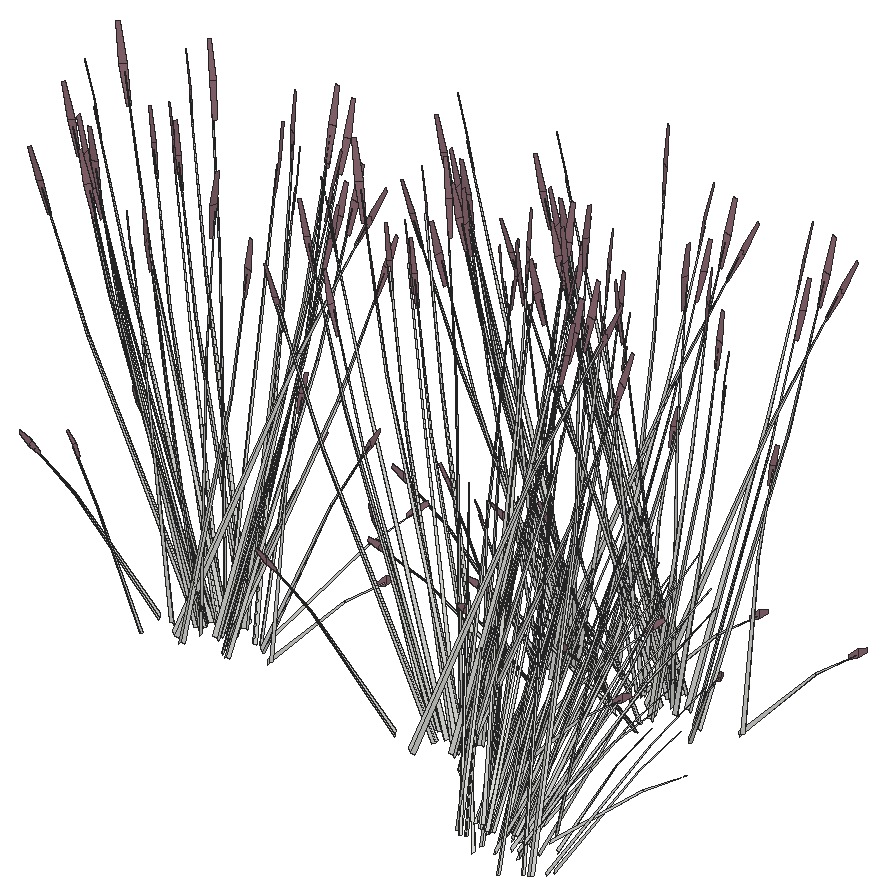
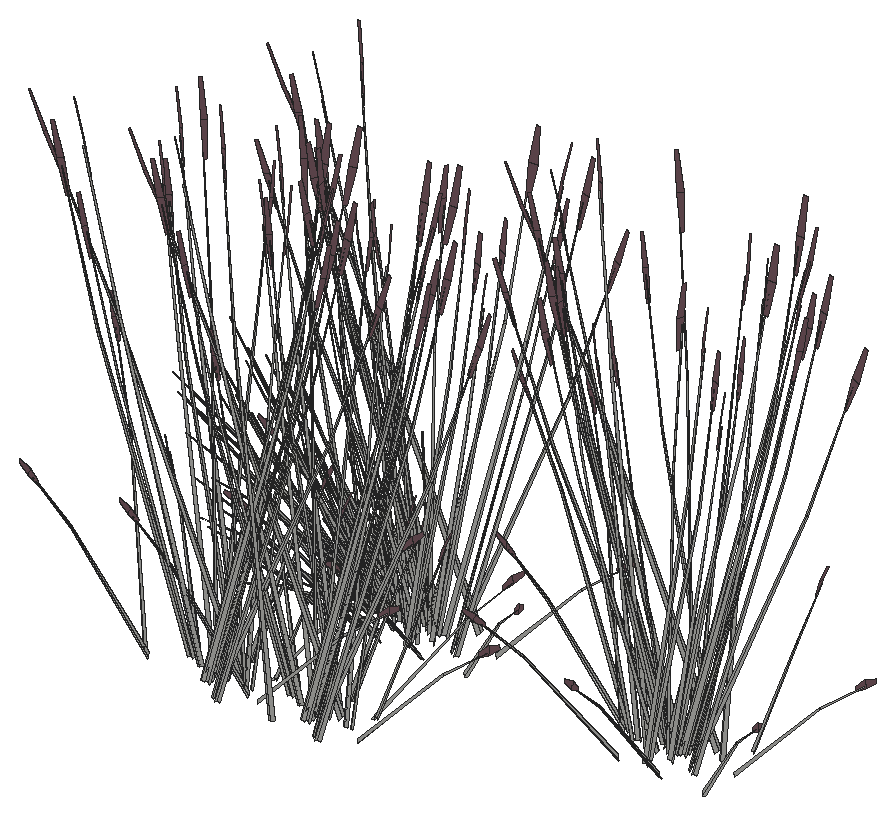
# SketchUp Ruby script. Lengths in inches.
U = 1.inch
M = Sketchup.active_model
def pt(a) = Geom::Point3d.new(a.map { |v| v * U })
def face(e, loops, mat)
  f = e.add_face(loops[0].map { |a| pt(a) })
  loops[1..].each { |l| e.add_face(l.map { |a| pt(a) }).erase! }
  f.material = f.back_material = mat if mat
  f
end
# faces: each face lists its corners as indices into pts; further lists are holes
def faces(e, pts, list, mat = nil) = list.each { |f| face(e, (f[0].is_a?(Array) ? f : [f]).map { |l| l.map { |i| pts[i] } }, mat) }
# xy, xz, yz: faces in a plane at the given z, y or x. An outline is a flat list of corners, or four numbers for a rectangle; further outlines are holes
def ring(l) = l.size == 4 ? [[l[0], l[1]], [l[2], l[1]], [l[2], l[3]], [l[0], l[3]]] : l.each_slice(2).to_a
def flat(e, list, mat, &to3) = list.each { |f| face(e, (f[0].is_a?(Array) ? f : [f]).map { |l| ring(l).map { |u, v| to3.(u, v) } }, mat) }
def xy(e, z, list, mat = nil) = flat(e, list, mat) { |x, y| [x, y, z] }
def xz(e, y, list, mat = nil) = flat(e, list, mat) { |x, z| [x, y, z] }
def yz(e, x, list, mat = nil) = flat(e, list, mat) { |y, z| [x, y, z] }
def lines(e, pts, list) = list.each { |a, b| e.add_line(pt(pts[a]), pt(pts[b])) }
# prism: a flat outline (further loops are holes) pulled along v
def prism(e, loops, v, mat = nil)
  f = face(e, loops, mat); d = Geom::Vector3d.new(v.map { |x| x * U })
  f.pushpull(f.normal.samedirection?(d) ? d.length : -d.length)
end
def box(e, o, s, mat = nil) = prism(e, [[o, [o[0] + s[0], o[1], o[2]], [o[0] + s[0], o[1] + s[1], o[2]], [o[0], o[1] + s[1], o[2]]]], [0, 0, s[2]], mat)
def at(x, y, z, deg = 0) = Geom::Transformation.translation(pt([x, y, z])) * Geom::Transformation.rotation(ORIGIN, Z_AXIS, deg.degrees)
def axes(o, x, y, z) = Geom::Transformation.new([*x, 0, *y, 0, *z, 0, *pt(o).to_a, 1])
def part(name) = M.definitions.add(name)
# library, detail: a bought-in or finely detailed component or shape, given as its bounding box
def library(name, o, s) = part(name).tap { |d| box(d.entities, o, s) }
def detail(e, o, s) = box(e.add_group.entities, o, s)
def put(e, d, t, mat = nil) = e.add_instance(d, t).tap { |i| i.material = mat if mat }
def group(e, t, mat = nil) = e.add_group.tap { |g| g.transformation = t; g.material = mat if mat }.entities
root = M.entities
M.materials.add("LightPink_Translucent").color = [144, 107, 117]
c1 = part("blade")
p = [[2.15,0.21,22],[0,0.17,0],[0.09,0.45,0],[2.18,0.31,22],[2.29,0.31,22],[0.38,0.45,0],
  [2.48,0.24,33],[2.49,0.24,33],[2.48,0.22,33]]
faces(c1.entities,p,[[0,1,2,3],[4,5,2,3],[6,3,4,7],[8,0,3,6]])
c2 = part("seeds")
p = [[0.3,-0.1,1.38],[-0.01,-0.03,1.59],[-0.01,-0.03,0.03],[0.14,-0.07,-0.07],[0.29,-0.03,3],[0.15,0.01,3.11]]
faces(c2.entities,p,[[0,1,2,3],[1,0,4,5]],"LightPink_Translucent")
c3 = part("blade with seeds")
put(c3.entities,c1,at(0,0,0))
put(c3.entities,c2,axes([2.4,0.25,30.99],[1.5799,-0.05474,1.17369],[-0.12525,1.92788,0.29478],[-0.07173,-0.02425,1.56792]))
c4 = part("blade with seeds\#1")
put(c4.entities,c1,at(0,0,0))
put(root,c3,axes([30.54,56.74,44.21],[0.59459,-0.93321,-0.44739],[1.23546,0.44912,0.21531],[0,-0.21512,1.43643]))
put(root,c3,axes([31.08,56.27,44.67],[-0.1428,-1.18174,-0.29095],[1.48733,-0.07145,-0.50002],[0.26191,-0.15741,1.59708]))
put(root,c4,axes([80.07,48.07,38.91],[-0.15413,-0.36483,1.28914],[0.46474,-0.90077,-0.27724],[0.40213,0.2681,0.55117]))
put(root,c3,axes([27.39,56.34,44.03],[0.85545,-0.64616,-0.30978],[0.85545,0.64616,0.30978],[0,-0.20813,1.38974]))
put(root,c3,axes([27.05,53.24,44.13],[-0.35352,0.84566,-0.03893],[-1.08806,-0.26014,-0.17649],[-0.1652,-0.13832,0.58215]))
put(root,c4,axes([71.29,48.59,38.49],[0.7978,0.33351,-0.03509],[-0.24541,1.02647,-0.15911],[-0.13049,0.15585,0.52479]))
put(root,c3,axes([61.53,54.7,44.06],[-1.27479,-0.1698,-0.62353],[0.26901,-1.04736,-0.16365],[-0.38043,-0.12691,1.37633]))
put(root,c3,axes([30.39,57.51,44.67],[-1.38012,-0.49416,-0.29095],[0.66454,-1.04299,-0.50002],[-0.04337,-0.25608,1.59708]))
put(root,c4,axes([76.27,48.65,41.13],[-0.13963,-1.00636,0.31925],[0.79822,-0.26574,-0.41216],[0.2144,0.28839,0.78863]))
put(root,c3,axes([30.88,53.66,44.03],[1.14332,0.25625,-0.30978],[-0.28787,0.90242,0.30978],[0.23049,-0.10406,1.38974]))
put(root,c3,axes([61.23,51.77,43.59],[-1.20625,0.41464,1.28929],[-0.38394,-1.1897,0.50096],[0.74071,0.01979,1.46642]))
put(root,c4,axes([78.54,50.93,41.66],[0.2608,-1.0202,-0.05849],[0.8027,0.31383,-0.26518],[0.12187,0.16686,0.87466]))
put(root,c4,axes([78.66,46.76,38.71],[0.97904,0.72283,0],[-0.54599,1.20931,-0.46523],[-0.12435,0.27543,1.47583]))
put(root,c4,axes([78.07,47.41,38.39],[-0.48852,1.08202,-0.44759],[-0.87598,-0.64674,0],[-0.11126,0.24644,1.41987]))
put(root,c3,axes([70.66,53.38,43.49],[-0.06405,-0.15723,1.76342],[0.44421,-0.91974,-0.26939],[0.4481,-0.01323,0.30037]))
put(root,c3,axes([57.43,53.22,43.49],[0.03108,0.16322,1.76342],[-0.62654,0.85237,-0.26939],[-0.44504,-0.04296,0.30037]))
put(root,c4,axes([71.57,45.96,41.0625],[-0.47225,0.98582,-0.64046],[-0.82754,-0.7006,0.07729],[-0.28197,0.35717,0.906]))
put(root,c4,axes([70.79,47.89,37.92],[0.12871,0.11199,1.5897],[0.2775,1.13173,-0.24285],[-0.25244,0.2734,0.27078]))
put(root,c4,axes([71.59,46.42,40.79],[0.23225,1.14083,-0.46065],[-0.87956,0.19957,-0.35681],[-0.25205,0.30642,0.88141]))
put(root,c4,axes([76.2,49.17,41.11],[0.53874,-1.06944,-0.10962],[0.78019,0.61612,-0.60845],[0.2712,0.30214,0.92453]))
put(root,c3,axes([60.18,56.3,44.03],[-0.28787,-0.90242,-0.30978],[1.14332,-0.25625,0.30978],[-0.23049,-0.10406,1.38974]))
put(root,c4,axes([76.2,45.84,38.43],[-0.16018,1.20264,-0.5621],[-0.98808,-0.25378,-0.14753],[-0.11973,0.3589,1.24074]))
put(root,c4,axes([70.81,45.62,41.47],[0.93666,0.77159,-0.12278],[-0.53962,1.11741,-0.68147],[-0.26463,0.38842,1.03548]))
put(root,c3,axes([64.36,52.38,44.67],[1.23732,-0.68758,-0.29095],[0.8228,0.97154,-0.50002],[0.30528,0.09867,1.59708]))
put(root,c4,axes([72.65,47.73,41.13],[0.61172,-0.65782,0.31925],[0.57907,0.75112,-0.41216],[-0.08811,0.38163,0.78863]))
put(root,c4,axes([72.09,48.32,40.84],[-0.74296,-0.05822,0.05797],[0.02037,-0.87906,0.45634],[-0.07774,0.33673,0.69585]))
put(root,c3,axes([59.86,56.68,44.02],[-1.14694,-0.51783,-0.49651],[0.68554,-0.92854,0],[-0.26122,-0.11794,1.57504]))
put(root,c3,axes([67.48,50.55,44.02],[1.14694,0.51783,-0.49651],[-0.68554,0.92854,0],[0.26122,0.11794,1.57504]))
put(root,c4,axes([78.4375,50.4,40.82],[0.19335,0.02874,1.57709],[0.67262,-0.81555,-0.24942],[0.31807,0.21351,0.12648]))
put(root,c3,axes([30.74,58.61,44.4375],[0.32481,-1.2272,-0.23429],[1.54007,0.21392,0.51271],[-0.26911,-0.16947,1.5644]))
put(root,c3,axes([62.98,54.85,44.67],[-1.23732,0.68758,-0.29095],[-0.8228,-0.97154,-0.50002],[-0.30528,-0.09867,1.59708]))
put(root,c4,axes([76.84,48.64,40.79],[0.89213,-0.297,-0.46065],[0.15606,1.12475,-0.35681],[0.23962,0.32232,0.88141]))
put(root,c4,axes([74.36,48.81,41.13],[0.27256,-0.96081,0.31925],[0.79518,0.28024,-0.41216],[0.07291,0.38684,0.78863]))
put(root,c4,axes([76.7,47.95,40.07],[-0.33582,-0.21526,1.54493],[0.69497,-0.90306,0.12492],[0.43315,0.40739,0.66044]))
put(root,c3,axes([67.16,50.9375,44.03],[0.28787,0.90242,-0.30978],[-1.14332,0.25625,0.30978],[0.23049,0.10406,1.38974]))
put(root,c4,axes([76.4,49.5625,40.84],[-0.4109,0.79368,0.05797],[-0.58514,-0.46209,0.45634],[0.18917,0.25446,0.69585]))
put(root,c4,axes([72.1,48.76,41.17],[-0.72104,-0.95477,0.48466],[0.76573,-0.82343,0.39963],[-0.133,0.44794,1.00289]))
put(root,c3,axes([30.63,58.11,44.21],[-0.73619,-0.86927,-0.44739],[1.11511,-0.61213,0.21531],[-0.23824,-0.10756,1.43643]))
put(root,c4,axes([76.57,49.34,40.84],[-0.89921,0.28673,0.43274],[-0.15606,-1.12475,0.35681],[0.21148,0.33149,0.89544]))
put(root,c3,axes([65.12,55.875,44.18],[1.2866,-0.3514,-0.19198],[0.45209,1.01223,0.00008],[0.14202,-0.03884,1.73897]))
put(root,c3,axes([38.23,57.77,43.98],[-0.7893,0.12429,1.41583],[-0.12563,-0.9893,0.08104],[0.55282,-0.14974,0.80566]))
put(root,c3,axes([39.67,56.89,44.26],[-0.75977,-0.66224,-0.06488],[0.83212,-0.6068,-0.29416],[0.23578,-0.04272,0.97024]))
put(root,c3,axes([65.8,52.53,44.06],[1.27479,0.1698,-0.62353],[-0.26901,1.04736,-0.16365],[0.38043,0.12691,1.37633]))
put(root,c4,axes([75.96,47.73,40.07],[-0.3002,-0.28876,1.54493],[0.81031,-0.72911,0.12492],[0.36902,0.50009,0.66044]))
put(root,c4,axes([79.11,50.02,37.92],[0.09761,-0.15508,1.5897],[0.90442,-0.26295,-0.24285],[0.19286,0.3437,0.27078]))
put(root,c4,axes([73.79,50.24,39.07],[-0.06991,-0.73811,1.03545],[0.616,0.4682,0.76078],[-0.09241,0.36475,0.22807]))
put(root,c3,axes([64.37,55.17,44.46],[-1.19666,-0.83357,-0.25192],[1.00694,-0.93603,0.5513],[-0.32224,0.09751,1.68216]))
put(root,c4,axes([72.33,48.66,40.65],[-0.61172,0.65782,-0.31925],[-0.57907,-0.75112,0.41216],[-0.08811,0.38163,0.78863]))
put(root,c4,axes([76.74,49.47,40.65],[0.13963,1.00636,-0.31925],[-0.79822,0.26574,0.41216],[0.2144,0.28839,0.78863]))
put(root,c4,axes([74.11,49.68,40.84],[-0.66618,0.42462,0.05797],[-0.32607,-0.77431,0.45634],[0.06434,0.34133,0.69585]))
put(root,c3,axes([29.97,58.44,44.06],[-1.27479,-0.1698,-0.62353],[0.26901,-1.04736,-0.16365],[-0.38043,-0.12691,1.37633]))
put(root,c4,axes([72.26,47.91,41.11],[0.99362,0.0619,-0.10962],[-0.02716,1.17208,-0.60845],[-0.06902,0.45141,0.92453]))
put(root,c4,axes([74.35,49.6,40.84],[-0.89085,-0.32663,0.43274],[0.30463,-1.07385,0.35681],[0.05354,0.4223,0.89544]))
put(root,c4,axes([74.1,49.21,41.11],[0.88471,-0.5817,-0.10962],[0.43476,1.03242,-0.60845],[0.11673,0.43507,0.92453]))
put(root,c4,axes([70.54,48.58,40.82],[-0.0069,0.24875,1.57709],[0.68965,0.79195,-0.24942],[-0.14092,0.42256,0.12648]))
put(root,c3,axes([65.14,52.87,44.21],[0.73619,0.86927,-0.44739],[-1.11511,0.61213,0.21531],[0.23824,0.10756,1.43643]))
put(root,c3,axes([29.67,55.51,43.59],[-1.20625,0.41464,1.28929],[-0.38394,-1.1897,0.50096],[0.74071,0.01979,1.46642]))
put(root,c4,axes([78.66,51.29,39.07],[-0.44281,-0.48182,1.03545],[0.70101,-0.19012,0.76078],[0.12552,0.34819,0.22807]))
put(root,c4,axes([71.12,49.53,40.82],[0.0975,-0.08571,1.59908],[0.87648,0.41319,-0.1511],[0.00634,0.41846,0.28298]))
put(root,c3,axes([39.09,57.125,43.49],[-0.06405,-0.15723,1.76342],[0.44421,-0.91974,-0.26939],[0.4481,-0.01323,0.30037]))
put(root,c3,axes([25.87,56.96,43.49],[0.03108,0.16322,1.76342],[-0.62654,0.85237,-0.26939],[-0.44504,-0.04296,0.30037]))
put(root,c4,axes([72.94,48.35,40.79],[0.6472,0.83949,-0.46065],[-0.68369,0.73521,-0.35681],[-0.09847,0.42653,0.88141]))
put(root,c4,axes([74.8,49.7,37.92],[0.15398,-0.02932,1.5897],[0.80412,0.59108,-0.24285],[-0.04053,0.41985,0.27078]))
put(root,c3,axes([28.61,60.04,44.03],[-0.28787,-0.90242,-0.30978],[1.14332,-0.25625,0.30978],[-0.23049,-0.10406,1.38974]))
put(root,c3,axes([63.76,54.99,44.21],[-1.33077,0.06393,-0.44739],[-0.12035,-1.06125,0.21531],[-0.23824,0.10756,1.43643]))
put(root,c4,axes([74.86,49.16,40.79],[0.88873,0.31321,-0.46065],[-0.30463,1.07385,-0.35681],[0.08149,0.43235,0.88141]))
put(root,c3,axes([32.8,56.12,44.67],[1.23732,-0.68758,-0.29095],[0.8228,0.97154,-0.50002],[0.30528,0.09867,1.59708]))
put(root,c4,axes([75.92,52.53,40.82],[0.0262,-0.14755,1.59908],[0.86326,-0.45644,-0.1511],[0.22658,0.30203,0.28298]))
put(root,c4,axes([74.45,49.82,40.65],[-0.27256,0.96081,-0.31925],[-0.79518,-0.28024,0.41216],[0.07291,0.38684,0.78863]))
put(root,c3,axes([28.3,60.43,44.02],[-1.14694,-0.51783,-0.49651],[0.68554,-0.92854,0],[-0.26122,-0.11794,1.57504]))
put(root,c3,axes([35.91,54.29,44.02],[1.14694,0.51783,-0.49651],[-0.68554,0.92854,0],[0.26122,0.11794,1.57504]))
put(root,c4,axes([72.09,48.49,40.07],[0.16834,-0.42944,1.54493],[0.70619,0.88871,0.12492],[-0.31858,0.5539,0.66044]))
put(root,c4,axes([72.73,47.97,41.0625],[-0.02352,1.1557,-0.64046],[-0.99061,-0.07762,0.07729],[-0.10454,0.48961,0.906]))
put(root,c4,axes([72.98,48.9,38.91],[0.27202,-0.22572,1.28914],[0.7394,0.52014,-0.27724],[-0.17673,0.53408,0.55117]))
put(root,c3,axes([31.41,58.6,44.67],[-1.23732,0.68758,-0.29095],[-0.8228,-0.97154,-0.50002],[-0.30528,-0.09867,1.59708]))
put(root,c4,axes([74.98,50.43,40.82],[0.12685,0.18879,1.57709],[0.92682,-0.01606,-0.24942],[0.12053,0.43275,0.12648]))
put(root,c3,axes([35.6,54.68,44.03],[0.28787,0.90242,-0.30978],[-1.14332,0.25625,0.30978],[0.23049,0.10406,1.38974]))
put(root,c4,axes([74.32,46.9,39.59],[-0.14134,-0.32863,1.5962],[0.98684,-0.11332,0.12492],[0.13095,0.71181,0.57049]))
put(root,c3,axes([33.56,59.62,44.18],[1.2866,-0.3514,-0.19198],[0.45209,1.01223,0.00008],[0.14202,-0.03884,1.73897]))
put(root,c3,axes([64.89,57.32,44.03],[-1.14332,-0.25625,-0.30978],[0.28787,-0.90242,0.30978],[-0.23049,0.10406,1.38974]))
put(root,c4,axes([76.94,50.45,38.91],[0.08021,-0.40179,1.28914],[0.81924,-0.25896,-0.27724],[0.15335,0.54576,0.55117]))
put(root,c4,axes([75.3125,49.2,40.07],[-0.20666,-0.40114,1.54493],[0.95496,-0.33772,0.12492],[0.21583,0.62976,0.66044]))
put(root,c3,axes([65.38,53.47,44.67],[1.38012,0.49416,-0.29095],[-0.66454,1.04299,-0.50002],[0.04337,0.25608,1.59708]))
put(root,c3,axes([34.24,56.28,44.06],[1.27479,0.1698,-0.62353],[-0.26901,1.04736,-0.16365],[0.38043,0.12691,1.37633]))
put(root,c3,axes([68.38,54.64,44.03],[-0.85545,0.64616,-0.30978],[-0.85545,-0.64616,0.30978],[0,0.20813,1.38974]))
put(root,c3,axes([64.69,54.7,44.67],[0.1428,1.18174,-0.29095],[-1.48733,0.07145,-0.50002],[-0.26191,0.15741,1.59708]))
put(root,c3,axes([32.8,58.91,44.46],[-1.19666,-0.83357,-0.25192],[1.00694,-0.93603,0.5513],[-0.32224,0.09751,1.68216]))
put(root,c3,axes([65.24,54.24,44.21],[-0.59459,0.93321,-0.44739],[-1.23546,-0.44912,0.21531],[0,0.21512,1.43643]))
put(root,c3,axes([33.58,56.61,44.21],[0.73619,0.86927,-0.44739],[-1.11511,0.61213,0.21531],[0.23824,0.10756,1.43643]))
put(root,c3,axes([63.8,55.61,44.06],[-0.82544,0.77843,-0.62353],[-1.0254,-0.70586,-0.16365],[-0.33076,0.19418,1.37633]))
put(root,c4,axes([73.625,49.4,40.07],[-0.02213,-0.47954,1.54493],[0.95907,0.31812,0.12492],[-0.05932,0.68338,0.66044]))
put(root,c3,axes([65.16,57.73,44.02],[-1.14694,0.51783,-0.49651],[-0.68554,-0.92854,0],[-0.26122,0.11794,1.57504]))
put(root,c3,axes([68.97,54.66,44.02],[0,1.03566,-0.49651],[-1.37109,0,0],[0,0.23588,1.57504]))
put(root,c3,axes([32.2,58.73,44.21],[-1.33077,0.06393,-0.44739],[-0.12035,-1.06125,0.21531],[-0.23824,0.10756,1.43643]))
put(root,c3,axes([67.42,57.92,43.49],[0.08928,-0.14952,1.76342],[1.12407,-0.44035,-0.26939],[0.34078,0.22791,0.30037]))
put(root,c3,axes([65.94,54.52,44.09],[0.44936,0.94823,-0.69212],[-1.29441,0.3415,-0.18165],[0.04967,0.32109,1.52773]))
put(root,c3,axes([57.1,57.79,43.49],[0.16438,0.10347,1.76342],[0.27873,0.95868,-0.26939],[-0.36432,0.20444,0.30037]))
put(root,c3,axes([63.03,68.4,43.49],[-0.20555,0.03731,1.76342],[-1.13672,-0.42002,-0.26939],[0.01907,-0.35034,0.30037]))
put(root,c3,axes([75.03,68.4,43.49],[-0.20555,0.03731,1.76342],[-1.13672,-0.42002,-0.26939],[0.01907,-0.35034,0.30037]))
put(root,c3,axes([33.33,61.0625,44.03],[-1.14332,-0.25625,-0.30978],[0.28787,-0.90242,0.30978],[-0.23049,0.10406,1.38974]))
put(root,c3,axes([33.82,57.21,44.67],[1.38012,0.49416,-0.29095],[-0.66454,1.04299,-0.50002],[0.04337,0.25608,1.59708]))
put(root,c3,axes([36.82,58.38,44.03],[-0.85545,0.64616,-0.30978],[-0.85545,-0.64616,0.30978],[0,0.20813,1.38974]))
put(root,c3,axes([33.13,58.45,44.67],[0.1428,1.18174,-0.29095],[-1.48733,0.07145,-0.50002],[-0.26191,0.15741,1.59708]))
put(root,c3,axes([33.67,57.98,44.21],[-0.59459,0.93321,-0.44739],[-1.23546,-0.44912,0.21531],[0,0.21512,1.43643]))
put(root,c3,axes([32.24,59.35,44.06],[-0.82544,0.77843,-0.62353],[-1.0254,-0.70586,-0.16365],[-0.33076,0.19418,1.37633]))
put(root,c3,axes([33.6,61.47,44.02],[-1.14694,0.51783,-0.49651],[-0.68554,-0.92854,0],[-0.26122,0.11794,1.57504]))
put(root,c3,axes([37.4,58.41,44.02],[0,1.03566,-0.49651],[-1.37109,0,0],[0,0.23588,1.57504]))
put(root,c3,axes([62.17,57.89,43.49],[0.19833,-0.05635,1.76342],[1.19302,0.31018,-0.26939],[0.03489,0.3496,0.30037]))
put(root,c3,axes([59.35,69.68,43.49],[-0.11871,0.13643,1.76342],[-1.19964,0.29415,-0.26939],[-0.2898,-0.26759,0.30037]))
put(root,c3,axes([71.35,69.68,43.49],[-0.11871,0.13643,1.76342],[-1.19964,0.29415,-0.26939],[-0.2898,-0.26759,0.30037]))
put(root,c3,axes([61.33,73.43,44.1],[-0.50328,-1.06202,-0.69835],[1.44974,-0.38248,-0.18329],[-0.05563,-0.35963,1.54149]))
put(root,c3,axes([73.33,73.43,44.1],[-0.50328,-1.06202,-0.69835],[1.44974,-0.38248,-0.18329],[-0.05563,-0.35963,1.54149]))
put(root,c3,axes([68.0625,70.1875,43.49],[-0.18342,-0.08159,1.76342],[-0.47115,-0.9115,-0.26939],[0.31784,-0.24736,0.30037]))
put(root,c3,axes([80.0625,70.1875,43.49],[-0.18342,-0.08159,1.76342],[-0.47115,-0.9115,-0.26939],[0.31784,-0.24736,0.30037]))
put(root,c3,axes([35.86,61.66,43.49],[0.08928,-0.14952,1.76342],[1.12407,-0.44035,-0.26939],[0.34078,0.22791,0.30037]))
put(root,c3,axes([34.37,58.27,44.09],[0.44936,0.94823,-0.69212],[-1.29441,0.3415,-0.18165],[0.04967,0.32109,1.52773]))
put(root,c3,axes([25.53,61.53,43.49],[0.16438,0.10347,1.76342],[0.27873,0.95868,-0.26939],[-0.36432,0.20444,0.30037]))
put(root,c3,axes([62.82,69.13,44.13],[-0.84686,0.59414,-0.03893],[-0.77596,-0.65071,-0.17649],[-0.05463,-0.18438,0.58215]))
put(root,c3,axes([74.82,69.13,44.13],[-0.84686,0.59414,-0.03893],[-0.77596,-0.65071,-0.17649],[-0.05463,-0.18438,0.58215]))
put(root,c3,axes([58.37,73.28,44.02],[0,-1.03566,-0.49651],[1.37109,0,0],[0,-0.23588,1.57504]))
put(root,c3,axes([70.37,73.28,44.02],[0,-1.03566,-0.49651],[1.37109,0,0],[0,-0.23588,1.57504]))
put(root,c3,axes([62.18,70.22,44.02],[1.14694,-0.51783,-0.49651],[0.68554,0.92854,0],[0.26122,-0.11794,1.57504]))
put(root,c3,axes([74.18,70.22,44.02],[1.14694,-0.51783,-0.49651],[0.68554,0.92854,0],[0.26122,-0.11794,1.57504]))
put(root,c3,axes([63.54,72.34,44.06],[0.82544,-0.77843,-0.62353],[1.0254,0.70586,-0.16365],[0.33076,-0.19418,1.37633]))
put(root,c3,axes([75.54,72.34,44.06],[0.82544,-0.77843,-0.62353],[1.0254,0.70586,-0.16365],[0.33076,-0.19418,1.37633]))
put(root,c3,axes([30.61,61.63,43.49],[0.19833,-0.05635,1.76342],[1.19302,0.31018,-0.26939],[0.03489,0.3496,0.30037]))
put(root,c3,axes([62.1,73.71,44.21],[0.59459,-0.93321,-0.44739],[1.23546,0.44912,0.21531],[0,-0.21512,1.43643]))
put(root,c3,axes([74.1,73.71,44.21],[0.59459,-0.93321,-0.44739],[1.23546,0.44912,0.21531],[0,-0.21512,1.43643]))
put(root,c3,axes([62.64,73.24,44.67],[-0.1428,-1.18174,-0.29095],[1.48733,-0.07145,-0.50002],[0.26191,-0.15741,1.59708]))
put(root,c3,axes([74.64,73.24,44.67],[-0.1428,-1.18174,-0.29095],[1.48733,-0.07145,-0.50002],[0.26191,-0.15741,1.59708]))
put(root,c3,axes([58.95,73.31,44.03],[0.85545,-0.64616,-0.30978],[0.85545,0.64616,0.30978],[0,-0.20813,1.38974]))
put(root,c3,axes([70.95,73.31,44.03],[0.85545,-0.64616,-0.30978],[0.85545,0.64616,0.30978],[0,-0.20813,1.38974]))
put(root,c3,axes([58.61,70.21,44.13],[-0.35352,0.84566,-0.03893],[-1.08806,-0.26014,-0.17649],[-0.1652,-0.13832,0.58215]))
put(root,c3,axes([70.61,70.21,44.13],[-0.35352,0.84566,-0.03893],[-1.08806,-0.26014,-0.17649],[-0.1652,-0.13832,0.58215]))
put(root,c3,axes([61.95,74.48,44.67],[-1.38012,-0.49416,-0.29095],[0.66454,-1.04299,-0.50002],[-0.04337,-0.25608,1.59708]))
put(root,c3,axes([73.95,74.48,44.67],[-1.38012,-0.49416,-0.29095],[0.66454,-1.04299,-0.50002],[-0.04337,-0.25608,1.59708]))
put(root,c3,axes([62.45,70.63,44.03],[1.14332,0.25625,-0.30978],[-0.28787,0.90242,0.30978],[0.23049,-0.10406,1.38974]))
put(root,c3,axes([74.45,70.63,44.03],[1.14332,0.25625,-0.30978],[-0.28787,0.90242,0.30978],[0.23049,-0.10406,1.38974]))
put(root,c3,axes([62.3,75.58,44.4375],[0.32481,-1.2272,-0.23429],[1.54007,0.21392,0.51271],[-0.26911,-0.16947,1.5644]))
put(root,c3,axes([74.3,75.58,44.4375],[0.32481,-1.2272,-0.23429],[1.54007,0.21392,0.51271],[-0.26911,-0.16947,1.5644]))
put(root,c3,axes([62.19,75.08,44.21],[-0.73619,-0.86927,-0.44739],[1.11511,-0.61213,0.21531],[-0.23824,-0.10756,1.43643]))
put(root,c3,axes([74.19,75.08,44.21],[-0.73619,-0.86927,-0.44739],[1.11511,-0.61213,0.21531],[-0.23824,-0.10756,1.43643]))
put(root,c3,axes([71.23,73.86,44.26],[-0.75977,-0.66224,-0.06488],[0.83212,-0.6068,-0.29416],[0.23578,-0.04272,0.97024]))
put(root,c3,axes([83.23,73.86,44.26],[-0.75977,-0.66224,-0.06488],[0.83212,-0.6068,-0.29416],[0.23578,-0.04272,0.97024]))
put(root,c3,axes([61.53,75.41,44.06],[-1.27479,-0.1698,-0.62353],[0.26901,-1.04736,-0.16365],[-0.38043,-0.12691,1.37633]))
put(root,c3,axes([73.53,75.41,44.06],[-1.27479,-0.1698,-0.62353],[0.26901,-1.04736,-0.16365],[-0.38043,-0.12691,1.37633]))
put(root,c3,axes([61.23,72.48,43.59],[-1.20625,0.41464,1.28929],[-0.38394,-1.1897,0.50096],[0.74071,0.01979,1.46642]))
put(root,c3,axes([73.23,72.48,43.59],[-1.20625,0.41464,1.28929],[-0.38394,-1.1897,0.50096],[0.74071,0.01979,1.46642]))
put(root,c3,axes([70.66,74.09,43.49],[-0.06405,-0.15723,1.76342],[0.44421,-0.91974,-0.26939],[0.4481,-0.01323,0.30037]))
put(root,c3,axes([82.66,74.09,43.49],[-0.06405,-0.15723,1.76342],[0.44421,-0.91974,-0.26939],[0.4481,-0.01323,0.30037]))
put(root,c3,axes([57.43,73.93,43.49],[0.03108,0.16322,1.76342],[-0.62654,0.85237,-0.26939],[-0.44504,-0.04296,0.30037]))
put(root,c3,axes([69.43,73.93,43.49],[0.03108,0.16322,1.76342],[-0.62654,0.85237,-0.26939],[-0.44504,-0.04296,0.30037]))
put(root,c3,axes([60.18,77.01,44.03],[-0.28787,-0.90242,-0.30978],[1.14332,-0.25625,0.30978],[-0.23049,-0.10406,1.38974]))
put(root,c3,axes([72.18,77.01,44.03],[-0.28787,-0.90242,-0.30978],[1.14332,-0.25625,0.30978],[-0.23049,-0.10406,1.38974]))
put(root,c3,axes([64.36,73.09,44.67],[1.23732,-0.68758,-0.29095],[0.8228,0.97154,-0.50002],[0.30528,0.09867,1.59708]))
put(root,c3,axes([76.36,73.09,44.67],[1.23732,-0.68758,-0.29095],[0.8228,0.97154,-0.50002],[0.30528,0.09867,1.59708]))
put(root,c3,axes([59.86,77.4,44.02],[-1.14694,-0.51783,-0.49651],[0.68554,-0.92854,0],[-0.26122,-0.11794,1.57504]))
put(root,c3,axes([71.86,77.4,44.02],[-1.14694,-0.51783,-0.49651],[0.68554,-0.92854,0],[-0.26122,-0.11794,1.57504]))
put(root,c3,axes([67.48,71.26,44.02],[1.14694,0.51783,-0.49651],[-0.68554,0.92854,0],[0.26122,0.11794,1.57504]))
put(root,c3,axes([79.48,71.26,44.02],[1.14694,0.51783,-0.49651],[-0.68554,0.92854,0],[0.26122,0.11794,1.57504]))
put(root,c3,axes([62.98,75.57,44.67],[-1.23732,0.68758,-0.29095],[-0.8228,-0.97154,-0.50002],[-0.30528,-0.09867,1.59708]))
put(root,c3,axes([74.98,75.57,44.67],[-1.23732,0.68758,-0.29095],[-0.8228,-0.97154,-0.50002],[-0.30528,-0.09867,1.59708]))
put(root,c3,axes([67.16,71.65,44.03],[0.28787,0.90242,-0.30978],[-1.14332,0.25625,0.30978],[0.23049,0.10406,1.38974]))
put(root,c3,axes([79.16,71.65,44.03],[0.28787,0.90242,-0.30978],[-1.14332,0.25625,0.30978],[0.23049,0.10406,1.38974]))
put(root,c3,axes([65.12,76.59,44.18],[1.2866,-0.3514,-0.19198],[0.45209,1.01223,0.00008],[0.14202,-0.03884,1.73897]))
